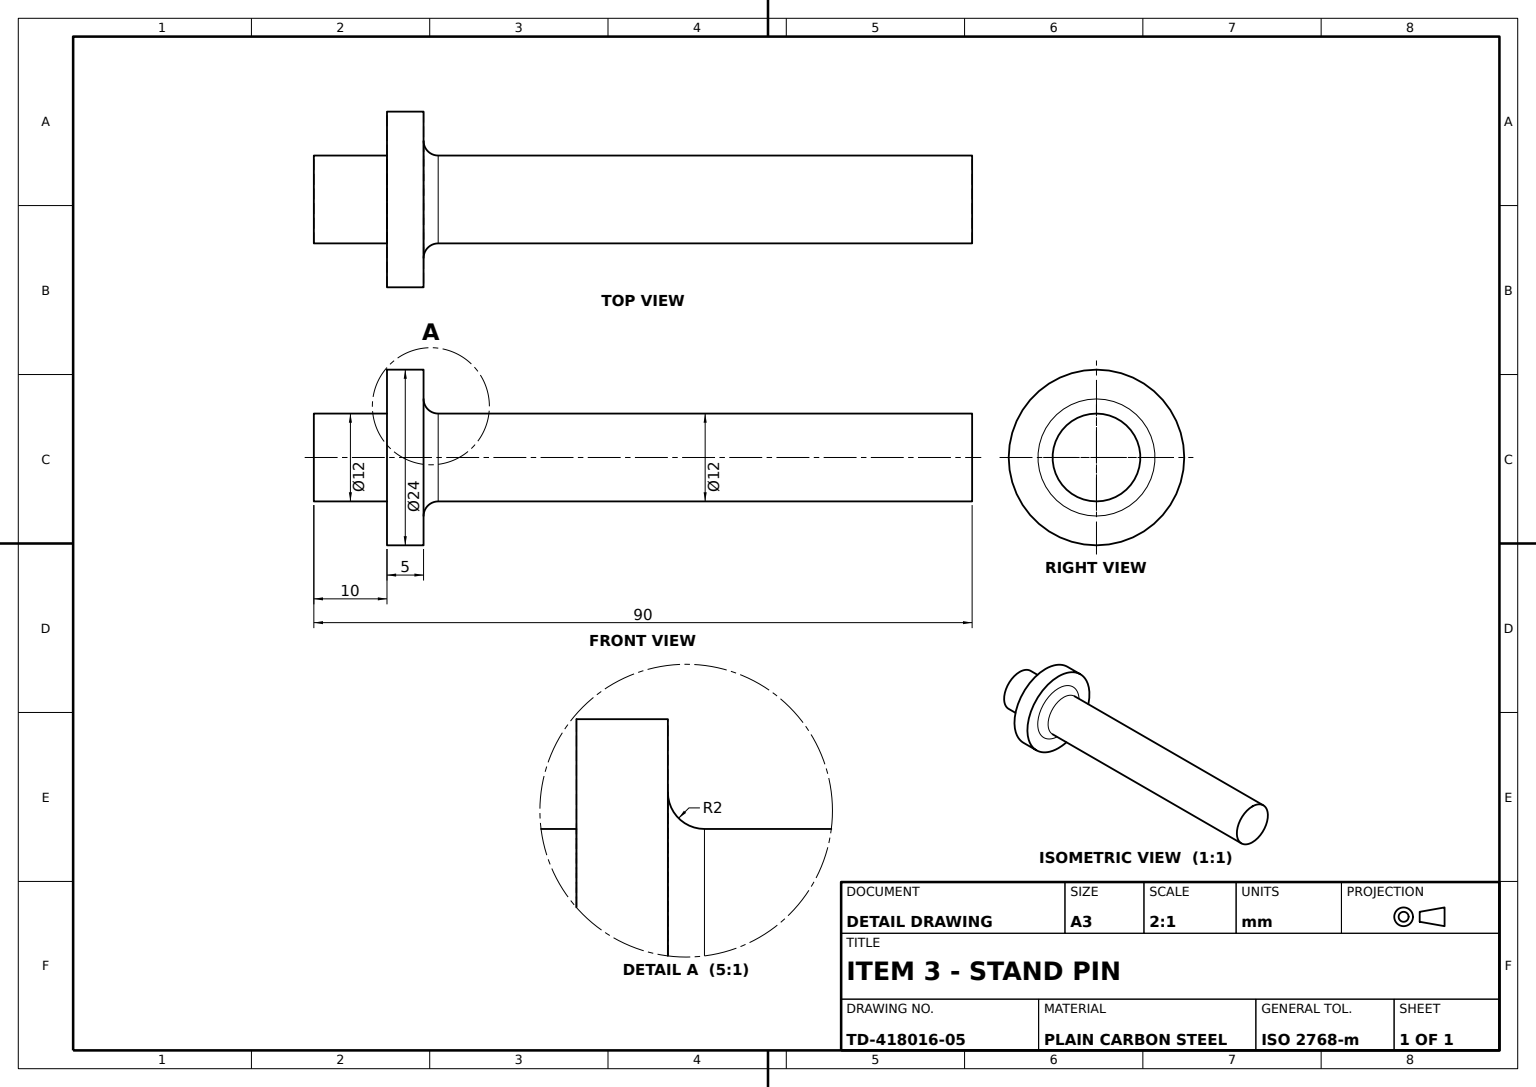
ISO-10303-21;
HEADER;
FILE_DESCRIPTION((''),'2;1');
FILE_NAME('','',(''),(''),'','','');
FILE_SCHEMA(('AUTOMOTIVE_DESIGN'));
ENDSEC;
DATA;
#1=APPLICATION_CONTEXT('');
#2=PRODUCT_CONTEXT('',#1,'mechanical');
#3=PRODUCT('','','',(#2));
#4=PRODUCT_DEFINITION_FORMATION('','',#3);
#5=PRODUCT_DEFINITION_CONTEXT('',#1,'design');
#6=PRODUCT_DEFINITION('','',#4,#5);
#7=PRODUCT_DEFINITION_SHAPE('','',#6);
#8=(LENGTH_UNIT()NAMED_UNIT(*)SI_UNIT(.MILLI.,.METRE.));
#9=(NAMED_UNIT(*)PLANE_ANGLE_UNIT()SI_UNIT($,.RADIAN.));
#10=(NAMED_UNIT(*)SI_UNIT($,.STERADIAN.)SOLID_ANGLE_UNIT());
#11=UNCERTAINTY_MEASURE_WITH_UNIT(LENGTH_MEASURE(1.E-05),#8,'distance_accuracy_value','');
#12=(GEOMETRIC_REPRESENTATION_CONTEXT(3)GLOBAL_UNCERTAINTY_ASSIGNED_CONTEXT((#11))GLOBAL_UNIT_ASSIGNED_CONTEXT((#8,#9,#10))REPRESENTATION_CONTEXT('',''));
#13=CARTESIAN_POINT('',(-6.,0.,0.));
#14=VERTEX_POINT('',#13);
#15=CARTESIAN_POINT('',(6.,0.,0.));
#16=VERTEX_POINT('',#15);
#17=CARTESIAN_POINT('',(0.,0.,0.));
#18=DIRECTION('',(0.,1.,0.));
#19=DIRECTION('',(-1.,0.,0.));
#20=AXIS2_PLACEMENT_3D('',#17,#18,#19);
#21=CIRCLE('',#20,6.);
#22=EDGE_CURVE('',#14,#16,#21,.T.);
#23=ORIENTED_EDGE('',*,*,#22,.F.);
#24=EDGE_CURVE('',#16,#14,#21,.T.);
#25=ORIENTED_EDGE('',*,*,#24,.F.);
#26=EDGE_LOOP('',(#23,#25));
#27=FACE_OUTER_BOUND('',#26,.T.);
#28=PLANE('',#20);
#29=ADVANCED_FACE('',(#27),#28,.F.);
#30=ORIENTED_EDGE('',*,*,#24,.T.);
#31=CARTESIAN_POINT('',(-6.,10.,0.));
#32=VERTEX_POINT('',#31);
#33=CARTESIAN_POINT('',(-6.,90.,0.));
#34=VECTOR('',#18,1000.);
#35=LINE('',#33,#34);
#36=EDGE_CURVE('',#14,#32,#35,.T.);
#37=ORIENTED_EDGE('',*,*,#36,.T.);
#38=CARTESIAN_POINT('',(6.,10.,0.));
#39=VERTEX_POINT('',#38);
#40=CARTESIAN_POINT('',(0.,10.,0.));
#41=AXIS2_PLACEMENT_3D('',#40,#18,#19);
#42=CIRCLE('',#41,6.);
#43=EDGE_CURVE('',#39,#32,#42,.T.);
#44=ORIENTED_EDGE('',*,*,#43,.F.);
#45=CARTESIAN_POINT('',(6.,90.,0.));
#46=LINE('',#45,#34);
#47=EDGE_CURVE('',#16,#39,#46,.T.);
#48=ORIENTED_EDGE('',*,*,#47,.F.);
#49=EDGE_LOOP('',(#30,#37,#44,#48));
#50=FACE_OUTER_BOUND('',#49,.T.);
#51=CARTESIAN_POINT('',(0.,90.,0.));
#52=AXIS2_PLACEMENT_3D('',#51,#18,#19);
#53=CYLINDRICAL_SURFACE('',#52,6.);
#54=ADVANCED_FACE('',(#50),#53,.T.);
#55=CARTESIAN_POINT('',(-12.,10.,0.));
#56=VERTEX_POINT('',#55);
#57=CARTESIAN_POINT('',(-12.,15.,0.));
#58=VERTEX_POINT('',#57);
#59=CARTESIAN_POINT('',(-12.,90.,0.));
#60=LINE('',#59,#34);
#61=EDGE_CURVE('',#56,#58,#60,.T.);
#62=ORIENTED_EDGE('',*,*,#61,.F.);
#63=CARTESIAN_POINT('',(12.,10.,0.));
#64=VERTEX_POINT('',#63);
#65=CIRCLE('',#41,12.);
#66=EDGE_CURVE('',#56,#64,#65,.T.);
#67=ORIENTED_EDGE('',*,*,#66,.T.);
#68=CARTESIAN_POINT('',(12.,15.,0.));
#69=VERTEX_POINT('',#68);
#70=CARTESIAN_POINT('',(12.,90.,0.));
#71=LINE('',#70,#34);
#72=EDGE_CURVE('',#64,#69,#71,.T.);
#73=ORIENTED_EDGE('',*,*,#72,.T.);
#74=CARTESIAN_POINT('',(0.,15.,0.));
#75=AXIS2_PLACEMENT_3D('',#74,#18,#19);
#76=CIRCLE('',#75,12.);
#77=EDGE_CURVE('',#58,#69,#76,.T.);
#78=ORIENTED_EDGE('',*,*,#77,.F.);
#79=EDGE_LOOP('',(#62,#67,#73,#78));
#80=FACE_OUTER_BOUND('',#79,.T.);
#81=CYLINDRICAL_SURFACE('',#52,12.);
#82=ADVANCED_FACE('',(#80),#81,.T.);
#83=CARTESIAN_POINT('',(6.,17.,0.));
#84=VERTEX_POINT('',#83);
#85=CARTESIAN_POINT('',(-6.,17.,0.));
#86=VERTEX_POINT('',#85);
#87=CARTESIAN_POINT('',(0.,17.,0.));
#88=DIRECTION('',(1.,0.,0.));
#89=AXIS2_PLACEMENT_3D('',#87,#18,#88);
#90=CIRCLE('',#89,6.);
#91=EDGE_CURVE('',#84,#86,#90,.T.);
#92=ORIENTED_EDGE('',*,*,#91,.F.);
#93=CARTESIAN_POINT('',(8.,15.,0.));
#94=VERTEX_POINT('',#93);
#95=CARTESIAN_POINT('',(8.,17.,0.));
#96=DIRECTION('',(0.,0.,-1.));
#97=AXIS2_PLACEMENT_3D('',#95,#96,#19);
#98=CIRCLE('',#97,2.);
#99=EDGE_CURVE('',#94,#84,#98,.T.);
#100=ORIENTED_EDGE('',*,*,#99,.F.);
#101=CARTESIAN_POINT('',(-8.,15.,0.));
#102=VERTEX_POINT('',#101);
#103=DIRECTION('',(0.,-1.,0.));
#104=AXIS2_PLACEMENT_3D('',#74,#103,#88);
#105=CIRCLE('',#104,8.);
#106=EDGE_CURVE('',#102,#94,#105,.T.);
#107=ORIENTED_EDGE('',*,*,#106,.F.);
#108=CARTESIAN_POINT('',(-8.,17.,0.));
#109=DIRECTION('',(0.,0.,1.));
#110=AXIS2_PLACEMENT_3D('',#108,#109,#88);
#111=CIRCLE('',#110,2.);
#112=EDGE_CURVE('',#102,#86,#111,.T.);
#113=ORIENTED_EDGE('',*,*,#112,.T.);
#114=EDGE_LOOP('',(#92,#100,#107,#113));
#115=FACE_OUTER_BOUND('',#114,.T.);
#116=AXIS2_PLACEMENT_3D('',#87,#103,#88);
#117=TOROIDAL_SURFACE('',#116,8.,2.);
#118=ADVANCED_FACE('',(#115),#117,.F.);
#119=VERTEX_POINT('',#33);
#120=EDGE_CURVE('',#86,#119,#35,.T.);
#121=ORIENTED_EDGE('',*,*,#120,.F.);
#122=EDGE_CURVE('',#86,#84,#90,.T.);
#123=ORIENTED_EDGE('',*,*,#122,.T.);
#124=VERTEX_POINT('',#45);
#125=EDGE_CURVE('',#84,#124,#46,.T.);
#126=ORIENTED_EDGE('',*,*,#125,.T.);
#127=CIRCLE('',#52,6.);
#128=EDGE_CURVE('',#119,#124,#127,.T.);
#129=ORIENTED_EDGE('',*,*,#128,.F.);
#130=EDGE_LOOP('',(#121,#123,#126,#129));
#131=FACE_OUTER_BOUND('',#130,.T.);
#132=ADVANCED_FACE('',(#131),#53,.T.);
#133=ORIENTED_EDGE('',*,*,#22,.T.);
#134=ORIENTED_EDGE('',*,*,#47,.T.);
#135=EDGE_CURVE('',#32,#39,#42,.T.);
#136=ORIENTED_EDGE('',*,*,#135,.F.);
#137=ORIENTED_EDGE('',*,*,#36,.F.);
#138=EDGE_LOOP('',(#133,#134,#136,#137));
#139=FACE_OUTER_BOUND('',#138,.T.);
#140=ADVANCED_FACE('',(#139),#53,.T.);
#141=EDGE_CURVE('',#64,#56,#65,.T.);
#142=ORIENTED_EDGE('',*,*,#141,.T.);
#143=ORIENTED_EDGE('',*,*,#61,.T.);
#144=EDGE_CURVE('',#69,#58,#76,.T.);
#145=ORIENTED_EDGE('',*,*,#144,.F.);
#146=ORIENTED_EDGE('',*,*,#72,.F.);
#147=EDGE_LOOP('',(#142,#143,#145,#146));
#148=FACE_OUTER_BOUND('',#147,.T.);
#149=ADVANCED_FACE('',(#148),#81,.T.);
#150=ORIENTED_EDGE('',*,*,#77,.T.);
#151=ORIENTED_EDGE('',*,*,#144,.T.);
#152=EDGE_LOOP('',(#150,#151));
#153=FACE_OUTER_BOUND('',#152,.T.);
#154=EDGE_CURVE('',#94,#102,#105,.T.);
#155=ORIENTED_EDGE('',*,*,#154,.T.);
#156=ORIENTED_EDGE('',*,*,#106,.T.);
#157=EDGE_LOOP('',(#155,#156));
#158=FACE_BOUND('',#157,.T.);
#159=CARTESIAN_POINT('',(6.,15.,0.));
#160=AXIS2_PLACEMENT_3D('',#159,#103,#88);
#161=PLANE('',#160);
#162=ADVANCED_FACE('',(#153,#158),#161,.F.);
#163=ORIENTED_EDGE('',*,*,#128,.T.);
#164=EDGE_CURVE('',#124,#119,#127,.T.);
#165=ORIENTED_EDGE('',*,*,#164,.T.);
#166=EDGE_LOOP('',(#163,#165));
#167=FACE_OUTER_BOUND('',#166,.T.);
#168=AXIS2_PLACEMENT_3D('',#45,#103,#88);
#169=PLANE('',#168);
#170=ADVANCED_FACE('',(#167),#169,.F.);
#171=ORIENTED_EDGE('',*,*,#66,.F.);
#172=ORIENTED_EDGE('',*,*,#141,.F.);
#173=EDGE_LOOP('',(#171,#172));
#174=FACE_OUTER_BOUND('',#173,.T.);
#175=ORIENTED_EDGE('',*,*,#135,.T.);
#176=ORIENTED_EDGE('',*,*,#43,.T.);
#177=EDGE_LOOP('',(#175,#176));
#178=FACE_BOUND('',#177,.T.);
#179=AXIS2_PLACEMENT_3D('',#63,#18,#19);
#180=PLANE('',#179);
#181=ADVANCED_FACE('',(#174,#178),#180,.F.);
#182=ORIENTED_EDGE('',*,*,#112,.F.);
#183=ORIENTED_EDGE('',*,*,#154,.F.);
#184=ORIENTED_EDGE('',*,*,#99,.T.);
#185=ORIENTED_EDGE('',*,*,#122,.F.);
#186=EDGE_LOOP('',(#182,#183,#184,#185));
#187=FACE_OUTER_BOUND('',#186,.T.);
#188=ADVANCED_FACE('',(#187),#117,.F.);
#189=ORIENTED_EDGE('',*,*,#91,.T.);
#190=ORIENTED_EDGE('',*,*,#120,.T.);
#191=ORIENTED_EDGE('',*,*,#164,.F.);
#192=ORIENTED_EDGE('',*,*,#125,.F.);
#193=EDGE_LOOP('',(#189,#190,#191,#192));
#194=FACE_OUTER_BOUND('',#193,.T.);
#195=ADVANCED_FACE('',(#194),#53,.T.);
#196=CLOSED_SHELL('',(#29,#54,#82,#118,#132,#140,#149,#162,#170,#181,#188,#195));
#197=MANIFOLD_SOLID_BREP('',#196);
#198=ADVANCED_BREP_SHAPE_REPRESENTATION('',(#197),#12);
#199=SHAPE_DEFINITION_REPRESENTATION(#7,#198);
ENDSEC;
END-ISO-10303-21;
